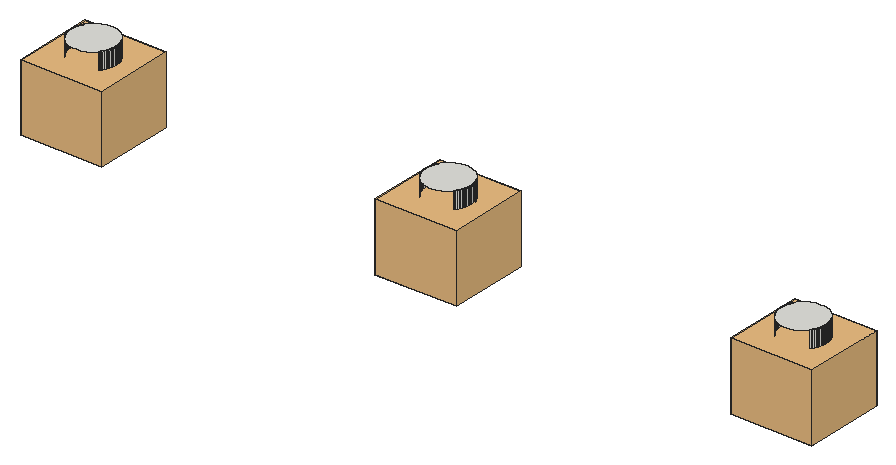
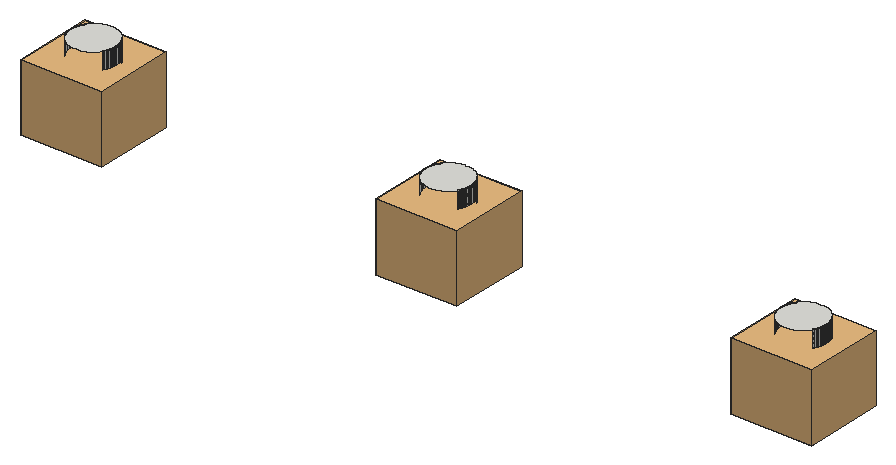
# SketchUp Ruby script. Lengths in inches.
U = 1.inch
M = Sketchup.active_model
def pt(a) = Geom::Point3d.new(a.map { |v| v * U })
def face(e, loops, mat)
  f = e.add_face(loops[0].map { |a| pt(a) })
  loops[1..].each { |l| e.add_face(l.map { |a| pt(a) }).erase! }
  f.material = f.back_material = mat if mat
  f
end
# faces: each face lists its corners as indices into pts; further lists are holes
def faces(e, pts, list, mat = nil) = list.each { |f| face(e, (f[0].is_a?(Array) ? f : [f]).map { |l| l.map { |i| pts[i] } }, mat) }
# xy, xz, yz: faces in a plane at the given z, y or x. An outline is a flat list of corners, or four numbers for a rectangle; further outlines are holes
def ring(l) = l.size == 4 ? [[l[0], l[1]], [l[2], l[1]], [l[2], l[3]], [l[0], l[3]]] : l.each_slice(2).to_a
def flat(e, list, mat, &to3) = list.each { |f| face(e, (f[0].is_a?(Array) ? f : [f]).map { |l| ring(l).map { |u, v| to3.(u, v) } }, mat) }
def xy(e, z, list, mat = nil) = flat(e, list, mat) { |x, y| [x, y, z] }
def xz(e, y, list, mat = nil) = flat(e, list, mat) { |x, z| [x, y, z] }
def yz(e, x, list, mat = nil) = flat(e, list, mat) { |y, z| [x, y, z] }
def lines(e, pts, list) = list.each { |a, b| e.add_line(pt(pts[a]), pt(pts[b])) }
# prism: a flat outline (further loops are holes) pulled along v
def prism(e, loops, v, mat = nil)
  f = face(e, loops, mat); d = Geom::Vector3d.new(v.map { |x| x * U })
  f.pushpull(f.normal.samedirection?(d) ? d.length : -d.length)
end
def box(e, o, s, mat = nil) = prism(e, [[o, [o[0] + s[0], o[1], o[2]], [o[0] + s[0], o[1] + s[1], o[2]], [o[0], o[1] + s[1], o[2]]]], [0, 0, s[2]], mat)
def at(x, y, z, deg = 0) = Geom::Transformation.translation(pt([x, y, z])) * Geom::Transformation.rotation(ORIGIN, Z_AXIS, deg.degrees)
def axes(o, x, y, z) = Geom::Transformation.new([*x, 0, *y, 0, *z, 0, *pt(o).to_a, 1])
def part(name) = M.definitions.add(name)
# library, detail: a bought-in or finely detailed component or shape, given as its bounding box
def library(name, o, s) = part(name).tap { |d| box(d.entities, o, s) }
def detail(e, o, s) = box(e.add_group.entities, o, s)
def put(e, d, t, mat = nil) = e.add_instance(d, t).tap { |i| i.material = mat if mat }
def group(e, t, mat = nil) = e.add_group.tap { |g| g.transformation = t; g.material = mat if mat }.entities
root = M.entities
c1 = library("2",[-3.42,-3.42,-12.15],[10.84,10.84,12.15])
xy(root,250,[[55.9,272.75,55.66,272.78,55.59,272.79,55.51,272.8,55.43,272.82,55.35,272.83,55.28,272.85,55.2,272.875,55.13,272.9,55.05,272.92,54.91,272.98,54.83,273.01,54.76,273.04,54.69,273.08,54.625,273.11,54.55,273.15,54.49,273.19,54.42,273.23,54.36,273.28,54.29,273.32,53.99,273.57,53.88,273.68,53.83,273.74,53.77,273.8,53.67,273.92,53.63,273.99,53.58,274.05,53.54,274.12,53.5,274.18,53.38,274.39,53.35,274.46,53.3125,274.53,53.28,274.6,53.25,274.67,53.23,274.75,53.2,274.82,53.18,274.9,53.16,274.97,53.14,275.05,53.12,275.125,53.11,275.2,53.09,275.28,53.08,275.36,53.07,275.4375,53.0625,275.51,53.06,275.59,53.06,275.67,53.05,275.75,53.06,275.83,53.06,275.91,53.0625,275.99,53.07,276.0625,53.08,276.14,53.09,276.22,53.11,276.3,53.12,276.375,53.14,276.45,53.16,276.53,53.18,276.6,53.2,276.68,53.23,276.75,53.25,276.83,53.28,276.9,53.3125,276.97,53.35,277.04,53.38,277.11,53.5,277.32,53.54,277.38,53.58,277.45,53.63,277.51,53.67,277.58,53.77,277.7,53.83,277.76,53.88,277.82,53.99,277.93,54.29,278.18,54.36,278.22,54.42,278.27,54.49,278.31,54.55,278.35,54.625,278.39,54.69,278.42,54.76,278.46,54.83,278.49,54.91,278.52,55.05,278.58,55.13,278.6,55.2,278.625,55.28,278.65,55.35,278.67,55.43,278.68,55.51,278.7,55.59,278.71,55.66,278.72,55.9,278.75,56.21,278.75,56.45,278.72,56.52,278.71,56.6,278.7,56.68,278.68,56.76,278.67,56.83,278.65,56.91,278.625,56.98,278.6,57.06,278.58,57.27,278.49,57.35,278.46,57.42,278.42,57.49,278.39,57.55,278.35,57.62,278.31,57.6875,278.27,57.75,278.22,57.82,278.18,58,278.03,58.0625,277.98,58.12,277.93,58.23,277.82,58.28,277.76,58.34,277.7,58.39,277.64,58.43,277.58,58.48,277.51,58.53,277.45,58.57,277.38,58.61,277.32,58.73,277.11,58.76,277.04,58.8,276.97,58.86,276.83,58.88,276.75,58.91,276.68,58.93,276.6,58.95,276.53,58.97,276.45,58.99,276.375,59,276.3,59.02,276.22,59.03,276.14,59.04,276.0625,59.05,275.99,59.05,275.51,59.04,275.4375,59.03,275.36,59.02,275.28,59,275.2,58.99,275.125,58.97,275.05,58.95,274.97,58.93,274.9,58.91,274.82,58.88,274.75,58.86,274.67,58.8,274.53,58.76,274.46,58.73,274.39,58.61,274.18,58.57,274.12,58.53,274.05,58.48,273.99,58.43,273.92,58.39,273.86,58.34,273.8,58.28,273.74,58.23,273.68,58.12,273.57,58.0625,273.52,58,273.47,57.82,273.32,57.75,273.28,57.6875,273.23,57.62,273.19,57.55,273.15,57.49,273.11,57.42,273.08,57.35,273.04,57.27,273.01,57.06,272.92,56.98,272.9,56.91,272.875,56.83,272.85,56.76,272.83,56.68,272.82,56.6,272.8,56.52,272.79,56.45,272.78,56.21,272.75],[103.34,272.75,103.26,272.76,103.1875,272.77,103.11,272.78,102.95,272.8,102.875,272.82,102.8,272.83,102.72,272.85,102.65,272.875,102.57,272.9,102.5,272.92,102.42,272.95,102.21,273.04,102.14,273.08,102.07,273.11,101.93,273.19,101.87,273.23,101.8,273.28,101.74,273.32,101.67,273.37,101.43,273.57,101.38,273.63,101.32,273.68,101.12,273.92,101.07,273.99,101.03,274.05,100.98,274.12,100.94,274.18,100.86,274.32,100.83,274.39,100.79,274.46,100.7,274.67,100.67,274.75,100.65,274.82,100.625,274.9,100.6,274.97,100.58,275.05,100.57,275.125,100.55,275.2,100.53,275.36,100.52,275.4375,100.51,275.51,100.5,275.59,100.5,275.91,100.51,275.99,100.52,276.0625,100.53,276.14,100.55,276.3,100.57,276.375,100.58,276.45,100.6,276.53,100.625,276.6,100.65,276.68,100.67,276.75,100.7,276.83,100.79,277.04,100.83,277.11,100.86,277.18,100.94,277.32,100.98,277.38,101.03,277.45,101.07,277.51,101.12,277.58,101.32,277.82,101.38,277.87,101.43,277.93,101.67,278.13,101.74,278.18,101.8,278.22,101.87,278.27,101.93,278.31,102.07,278.39,102.14,278.42,102.21,278.46,102.42,278.55,102.5,278.58,102.57,278.6,102.65,278.625,102.72,278.65,102.8,278.67,102.875,278.68,102.95,278.7,103.11,278.72,103.1875,278.73,103.26,278.74,103.34,278.75,103.66,278.75,103.74,278.74,103.8125,278.73,103.89,278.72,104.05,278.7,104.125,278.68,104.2,278.67,104.28,278.65,104.35,278.625,104.43,278.6,104.5,278.58,104.58,278.55,104.79,278.46,104.86,278.42,104.93,278.39,105.07,278.31,105.13,278.27,105.2,278.22,105.26,278.18,105.33,278.13,105.57,277.93,105.62,277.87,105.68,277.82,105.88,277.58,105.93,277.51,105.97,277.45,106.02,277.38,106.06,277.32,106.14,277.18,106.17,277.11,106.21,277.04,106.3,276.83,106.33,276.75,106.35,276.68,106.375,276.6,106.4,276.53,106.42,276.45,106.43,276.375,106.45,276.3,106.47,276.14,106.48,276.0625,106.49,275.99,106.5,275.91,106.5,275.59,106.49,275.51,106.48,275.4375,106.47,275.36,106.45,275.2,106.43,275.125,106.42,275.05,106.4,274.97,106.375,274.9,106.35,274.82,106.33,274.75,106.3,274.67,106.21,274.46,106.17,274.39,106.14,274.32,106.06,274.18,106.02,274.12,105.97,274.05,105.93,273.99,105.88,273.92,105.68,273.68,105.62,273.63,105.57,273.57,105.33,273.37,105.26,273.32,105.2,273.28,105.13,273.23,105.07,273.19,104.93,273.11,104.86,273.08,104.79,273.04,104.58,272.95,104.5,272.92,104.43,272.9,104.35,272.875,104.28,272.85,104.2,272.83,104.125,272.82,104.05,272.8,103.89,272.78,103.8125,272.77,103.74,272.76,103.66,272.75],[150.79,272.75,150.55,272.78,150.48,272.79,150.4,272.8,150.32,272.82,150.24,272.83,150.17,272.85,150.09,272.875,150.02,272.9,149.94,272.92,149.73,273.01,149.65,273.04,149.58,273.08,149.51,273.11,149.45,273.15,149.38,273.19,149.3125,273.23,149.25,273.28,149.18,273.32,149,273.47,148.9375,273.52,148.88,273.57,148.77,273.68,148.72,273.74,148.66,273.8,148.61,273.86,148.57,273.92,148.52,273.99,148.47,274.05,148.43,274.12,148.39,274.18,148.27,274.39,148.24,274.46,148.2,274.53,148.14,274.67,148.12,274.75,148.09,274.82,148.07,274.9,148.05,274.97,148.03,275.05,148.01,275.125,148,275.2,147.98,275.28,147.97,275.36,147.96,275.4375,147.95,275.51,147.95,275.99,147.96,276.0625,147.97,276.14,147.98,276.22,148,276.3,148.01,276.375,148.03,276.45,148.05,276.53,148.07,276.6,148.09,276.68,148.12,276.75,148.14,276.83,148.2,276.97,148.24,277.04,148.27,277.11,148.39,277.32,148.43,277.38,148.47,277.45,148.52,277.51,148.57,277.58,148.61,277.64,148.66,277.7,148.72,277.76,148.77,277.82,148.88,277.93,148.9375,277.98,149,278.03,149.18,278.18,149.25,278.22,149.3125,278.27,149.38,278.31,149.45,278.35,149.51,278.39,149.58,278.42,149.65,278.46,149.73,278.49,149.94,278.58,150.02,278.6,150.09,278.625,150.17,278.65,150.24,278.67,150.32,278.68,150.4,278.7,150.48,278.71,150.55,278.72,150.79,278.75,151.1,278.75,151.34,278.72,151.41,278.71,151.49,278.7,151.57,278.68,151.65,278.67,151.72,278.65,151.8,278.625,151.87,278.6,151.95,278.58,152.09,278.52,152.17,278.49,152.24,278.46,152.31,278.42,152.375,278.39,152.45,278.35,152.51,278.31,152.58,278.27,152.64,278.22,152.71,278.18,153.01,277.93,153.12,277.82,153.17,277.76,153.23,277.7,153.33,277.58,153.37,277.51,153.42,277.45,153.46,277.38,153.5,277.32,153.62,277.11,153.65,277.04,153.6875,276.97,153.72,276.9,153.75,276.83,153.77,276.75,153.8,276.68,153.82,276.6,153.84,276.53,153.86,276.45,153.88,276.375,153.89,276.3,153.91,276.22,153.92,276.14,153.93,276.0625,153.9375,275.99,153.94,275.91,153.94,275.83,153.95,275.75,153.94,275.67,153.94,275.59,153.9375,275.51,153.93,275.4375,153.92,275.36,153.91,275.28,153.89,275.2,153.88,275.125,153.86,275.05,153.84,274.97,153.82,274.9,153.8,274.82,153.77,274.75,153.75,274.67,153.72,274.6,153.6875,274.53,153.65,274.46,153.62,274.39,153.5,274.18,153.46,274.12,153.42,274.05,153.37,273.99,153.33,273.92,153.23,273.8,153.17,273.74,153.12,273.68,153.01,273.57,152.71,273.32,152.64,273.28,152.58,273.23,152.51,273.19,152.45,273.15,152.375,273.11,152.31,273.08,152.24,273.04,152.17,273.01,152.09,272.98,151.95,272.92,151.87,272.9,151.8,272.875,151.72,272.85,151.65,272.83,151.57,272.82,151.49,272.8,151.41,272.79,151.34,272.78,151.1,272.75]])
yz(root,53.06,[[275.59,247,275.67,250],[275.83,247,275.91,250]])
yz(root,59.05,[[275.51,247,275.59,250],[275.59,247,275.67,250],[275.67,247,275.75,250],[275.75,247,275.83,250],[275.83,247,275.91,250],
  [275.91,247,275.99,250]])
yz(root,100.5,[[275.59,247,275.67,250],[275.67,247,275.75,250],[275.75,247,275.83,250],[275.83,247,275.91,250]])
yz(root,106.5,[[275.59,247,275.67,250],[275.67,247,275.75,250],[275.75,247,275.83,250],[275.83,247,275.91,250]])
yz(root,147.95,[[275.51,247,275.59,250],[275.59,247,275.67,250],[275.67,247,275.75,250],[275.75,247,275.83,250],[275.83,247,275.91,250],
  [275.91,247,275.99,250]])
yz(root,153.94,[[275.59,247,275.67,250],[275.83,247,275.91,250]])
p = [[58.39,273.86,250],[58.39,273.86,247],[58.34,273.8,247],[58.34,273.8,250],[105.83,273.86,250],[105.83,273.86,247],
  [105.78,273.8,247],[105.78,273.8,250],[53.67,273.92,250],[53.67,273.92,247],[53.63,273.99,247],[53.63,273.99,250],
  [53.72,273.86,250],[53.72,273.86,247],[58.43,273.92,250],[58.43,273.92,247],[58.48,273.99,250],[58.48,273.99,247],
  [101.17,273.86,250],[101.17,273.86,247],[101.12,273.92,247],[101.12,273.92,250],[101.07,273.99,247],[101.07,273.99,250],
  [105.88,273.92,250],[105.88,273.92,247],[105.93,273.99,250],[105.93,273.99,247],[148.57,273.92,250],[148.57,273.92,247],
  [148.52,273.99,247],[148.52,273.99,250],[148.61,273.86,250],[148.61,273.86,247],[153.33,273.92,250],[153.33,273.92,247],
  [153.28,273.86,247],[153.28,273.86,250],[153.37,273.99,250],[153.37,273.99,247],[53.58,274.05,247],[53.58,274.05,250],
  [58.53,274.05,250],[58.53,274.05,247],[101.03,274.05,247],[101.03,274.05,250],[105.97,274.05,250],[105.97,274.05,247],
  [148.47,274.05,247],[148.47,274.05,250],[153.42,274.05,250],[153.42,274.05,247],[53.54,274.12,247],[53.54,274.12,250],
  [53.5,274.18,247],[53.5,274.18,250],[58.57,274.12,250],[58.57,274.12,247],[58.61,274.18,250],[58.61,274.18,247],
  [100.98,274.12,250],[100.98,274.12,247],[100.94,274.18,247],[100.94,274.18,250],[106.02,274.12,250],[106.02,274.12,247],
  [106.06,274.18,250],[106.06,274.18,247],[148.43,274.12,247],[148.43,274.12,250],[148.39,274.18,247],[148.39,274.18,250],
  [153.46,274.12,250],[153.46,274.12,247],[153.5,274.18,250],[153.5,274.18,247],[53.46,274.25,247],[53.46,274.25,250],
  [58.65,274.25,250],[58.65,274.25,247],[100.9,274.25,247],[100.9,274.25,250],[106.1,274.25,250],[106.1,274.25,247],
  [148.35,274.25,247],[148.35,274.25,250],[153.54,274.25,250],[153.54,274.25,247],[53.42,274.32,247],[53.42,274.32,250],
  [53.38,274.39,247],[53.38,274.39,250],[58.69,274.32,250],[58.69,274.32,247],[58.73,274.39,250],[58.73,274.39,247],
  [100.86,274.32,250],[100.86,274.32,247],[100.83,274.39,247],[100.83,274.39,250],[106.14,274.32,250],[106.14,274.32,247],
  [106.17,274.39,250],[106.17,274.39,247],[148.31,274.32,247],[148.31,274.32,250],[148.27,274.39,247],[148.27,274.39,250],
  [153.58,274.32,250],[153.58,274.32,247],[153.62,274.39,250],[153.62,274.39,247],[53.35,274.46,247],[53.35,274.46,250],
  [58.76,274.46,250],[58.76,274.46,247],[100.79,274.46,247],[100.79,274.46,250],[106.21,274.46,250],[106.21,274.46,247],
  [148.24,274.46,247],[148.24,274.46,250],[153.65,274.46,250],[153.65,274.46,247],[53.3125,274.53,247],[53.3125,274.53,250],
  [53.28,274.6,247],[53.28,274.6,250],[58.8,274.53,250],[58.8,274.53,247],[58.83,274.6,250],[58.83,274.6,247],
  [100.76,274.53,250],[100.76,274.53,247],[100.73,274.6,247],[100.73,274.6,250],[106.24,274.53,250],[106.24,274.53,247],
  [106.27,274.6,250],[106.27,274.6,247],[148.2,274.53,247],[148.2,274.53,250],[148.17,274.6,247],[148.17,274.6,250],
  [153.6875,274.53,250],[153.6875,274.53,247],[153.72,274.6,250],[153.72,274.6,247],[53.25,274.67,247],[53.25,274.67,250],
  [58.86,274.67,250],[58.86,274.67,247],[100.7,274.67,247],[100.7,274.67,250],[106.3,274.67,250],[106.3,274.67,247],
  [148.14,274.67,247],[148.14,274.67,250],[153.75,274.67,250],[153.75,274.67,247],[53.23,274.75,247],[53.23,274.75,250],
  [53.2,274.82,247],[53.2,274.82,250],[58.88,274.75,250],[58.88,274.75,247],[58.91,274.82,250],[58.91,274.82,247],
  [100.67,274.75,250],[100.67,274.75,247],[100.65,274.82,247],[100.65,274.82,250],[106.33,274.75,250],[106.33,274.75,247],
  [106.35,274.82,250],[106.35,274.82,247],[148.12,274.75,247],[148.12,274.75,250],[148.09,274.82,247],[148.09,274.82,250],
  [153.77,274.75,250],[153.77,274.75,247],[153.8,274.82,250],[153.8,274.82,247],[53.18,274.9,247],[53.18,274.9,250],
  [58.93,274.9,250],[58.93,274.9,247],[100.625,274.9,247],[100.625,274.9,250],[106.375,274.9,250],[106.375,274.9,247],
  [148.07,274.9,247],[148.07,274.9,250],[153.82,274.9,250],[153.82,274.9,247],[53.16,274.97,247],[53.16,274.97,250],
  [58.95,274.97,250],[58.95,274.97,247],[100.6,274.97,247],[100.6,274.97,250],[106.4,274.97,250],[106.4,274.97,247],
  [148.05,274.97,247],[148.05,274.97,250],[153.84,274.97,250],[153.84,274.97,247],[53.14,275.05,247],[53.14,275.05,250],
  [53.12,275.125,247],[53.12,275.125,250],[58.97,275.05,250],[58.97,275.05,247],[58.99,275.125,250],[58.99,275.125,247],
  [100.58,275.05,247],[100.58,275.05,250],[100.57,275.125,247],[100.57,275.125,250],[106.42,275.05,250],[106.42,275.05,247],
  [106.43,275.125,250],[106.43,275.125,247],[148.03,275.05,247],[148.03,275.05,250],[148.01,275.125,247],[148.01,275.125,250],
  [153.86,275.05,250],[153.86,275.05,247],[153.88,275.125,250],[153.88,275.125,247],[53.11,275.2,247],[53.11,275.2,250],
  [59,275.2,250],[59,275.2,247],[100.55,275.2,247],[100.55,275.2,250],[106.45,275.2,250],[106.45,275.2,247],
  [148,275.2,247],[148,275.2,250],[153.89,275.2,250],[153.89,275.2,247],[53.09,275.28,247],[53.09,275.28,250],
  [59.02,275.28,250],[59.02,275.28,247],[100.54,275.28,247],[100.54,275.28,250],[106.46,275.28,250],[106.46,275.28,247],
  [147.98,275.28,247],[147.98,275.28,250],[153.91,275.28,250],[153.91,275.28,247],[53.08,275.36,247],[53.08,275.36,250],
  [59.03,275.36,250],[59.03,275.36,247],[100.53,275.36,247],[100.53,275.36,250],[106.47,275.36,250],[106.47,275.36,247],
  [147.97,275.36,247],[147.97,275.36,250],[153.92,275.36,250],[153.92,275.36,247],[53.07,275.4375,247],[53.07,275.4375,250],
  [53.0625,275.51,247],[53.0625,275.51,250],[59.04,275.4375,250],[59.04,275.4375,247],[59.05,275.51,250],[59.05,275.51,247],
  [100.52,275.4375,247],[100.52,275.4375,250],[100.51,275.51,247],[100.51,275.51,250],[106.48,275.4375,250],[106.48,275.4375,247],
  [106.49,275.51,250],[106.49,275.51,247],[147.96,275.4375,247],[147.96,275.4375,250],[147.95,275.51,247],[147.95,275.51,250],
  [153.93,275.4375,250],[153.93,275.4375,247],[153.9375,275.51,250],[153.9375,275.51,247],[53.06,275.59,247],[53.06,275.59,250],
  [100.5,275.59,247],[100.5,275.59,250],[106.5,275.59,250],[106.5,275.59,247],[153.94,275.59,250],[153.94,275.59,247],
  [53.06,275.67,250],[53.06,275.67,247],[53.05,275.75,247],[53.05,275.75,250],[153.95,275.75,250],[153.95,275.75,247],
  [153.94,275.67,247],[153.94,275.67,250],[53.06,275.83,247],[53.06,275.83,250],[153.94,275.83,250],[153.94,275.83,247],
  [53.06,275.91,250],[53.06,275.91,247],[53.0625,275.99,247],[53.0625,275.99,250],[100.5,275.91,250],[100.5,275.91,247],
  [100.51,275.99,247],[100.51,275.99,250],[106.49,275.99,250],[106.49,275.99,247],[106.5,275.91,247],[106.5,275.91,250],
  [153.9375,275.99,250],[153.9375,275.99,247],[153.94,275.91,247],[153.94,275.91,250],[53.07,276.0625,247],[53.07,276.0625,250],
  [59.04,276.0625,250],[59.04,276.0625,247],[59.05,275.99,247],[59.05,275.99,250],[100.52,276.0625,247],[100.52,276.0625,250],
  [106.48,276.0625,250],[106.48,276.0625,247],[147.95,275.99,250],[147.95,275.99,247],[147.96,276.0625,247],[147.96,276.0625,250],
  [153.93,276.0625,250],[153.93,276.0625,247],[53.08,276.14,247],[53.08,276.14,250],[53.09,276.22,247],[53.09,276.22,250],
  [59.03,276.14,250],[59.03,276.14,247],[59.02,276.22,250],[59.02,276.22,247],[100.53,276.14,247],[100.53,276.14,250],
  [100.54,276.22,247],[100.54,276.22,250],[106.47,276.14,250],[106.47,276.14,247],[106.46,276.22,250],[106.46,276.22,247],
  [147.97,276.14,247],[147.97,276.14,250],[147.98,276.22,247],[147.98,276.22,250],[153.92,276.14,250],[153.92,276.14,247],
  [153.91,276.22,250],[153.91,276.22,247],[53.11,276.3,247],[53.11,276.3,250],[59,276.3,250],[59,276.3,247],
  [100.55,276.3,247],[100.55,276.3,250],[106.45,276.3,250],[106.45,276.3,247],[148,276.3,247],[148,276.3,250],
  [153.89,276.3,250],[153.89,276.3,247],[53.12,276.375,247],[53.12,276.375,250],[58.99,276.375,250],[58.99,276.375,247],
  [100.57,276.375,247],[100.57,276.375,250],[106.43,276.375,250],[106.43,276.375,247],[148.01,276.375,247],[148.01,276.375,250],
  [153.88,276.375,250],[153.88,276.375,247],[53.14,276.45,247],[53.14,276.45,250],[58.97,276.45,250],[58.97,276.45,247],
  [100.58,276.45,247],[100.58,276.45,250],[106.42,276.45,250],[106.42,276.45,247],[148.03,276.45,247],[148.03,276.45,250],
  [153.86,276.45,250],[153.86,276.45,247],[53.16,276.53,247],[53.16,276.53,250],[53.18,276.6,247],[53.18,276.6,250],
  [58.93,276.6,250],[58.93,276.6,247],[58.95,276.53,247],[58.95,276.53,250],[100.6,276.53,247],[100.6,276.53,250],
  [100.625,276.6,247],[100.625,276.6,250],[106.4,276.53,250],[106.4,276.53,247],[106.375,276.6,250],[106.375,276.6,247],
  [148.05,276.53,247],[148.05,276.53,250],[148.07,276.6,247],[148.07,276.6,250],[153.84,276.53,250],[153.84,276.53,247],
  [153.82,276.6,250],[153.82,276.6,247],[53.2,276.68,247],[53.2,276.68,250],[58.91,276.68,250],[58.91,276.68,247],
  [100.65,276.68,247],[100.65,276.68,250],[106.35,276.68,250],[106.35,276.68,247],[148.09,276.68,247],[148.09,276.68,250],
  [153.8,276.68,250],[153.8,276.68,247],[53.23,276.75,247],[53.23,276.75,250],[58.88,276.75,250],[58.88,276.75,247],
  [100.67,276.75,247],[100.67,276.75,250],[106.33,276.75,250],[106.33,276.75,247],[148.12,276.75,247],[148.12,276.75,250],
  [153.77,276.75,250],[153.77,276.75,247],[53.25,276.83,247],[53.25,276.83,250],[53.28,276.9,247],[53.28,276.9,250],
  [58.83,276.9,250],[58.83,276.9,247],[58.86,276.83,247],[58.86,276.83,250],[100.7,276.83,247],[100.7,276.83,250],
  [100.73,276.9,247],[100.73,276.9,250],[106.3,276.83,250],[106.3,276.83,247],[106.27,276.9,250],[106.27,276.9,247],
  [148.14,276.83,247],[148.14,276.83,250],[148.17,276.9,247],[148.17,276.9,250],[153.75,276.83,250],[153.75,276.83,247],
  [153.72,276.9,250],[153.72,276.9,247],[53.3125,276.97,247],[53.3125,276.97,250],[58.8,276.97,250],[58.8,276.97,247],
  [100.76,276.97,247],[100.76,276.97,250],[106.24,276.97,250],[106.24,276.97,247],[148.2,276.97,247],[148.2,276.97,250],
  [153.6875,276.97,250],[153.6875,276.97,247],[53.35,277.04,247],[53.35,277.04,250],[53.38,277.11,247],[53.38,277.11,250],
  [58.73,277.11,250],[58.73,277.11,247],[58.76,277.04,247],[58.76,277.04,250],[100.79,277.04,247],[100.79,277.04,250],
  [100.83,277.11,247],[100.83,277.11,250],[106.21,277.04,250],[106.21,277.04,247],[106.17,277.11,250],[106.17,277.11,247],
  [148.24,277.04,247],[148.24,277.04,250],[148.27,277.11,247],[148.27,277.11,250],[153.62,277.11,250],[153.62,277.11,247],
  [153.65,277.04,247],[153.65,277.04,250],[53.42,277.18,247],[53.42,277.18,250],[58.69,277.18,250],[58.69,277.18,247],
  [100.86,277.18,247],[100.86,277.18,250],[106.14,277.18,250],[106.14,277.18,247],[148.31,277.18,247],[148.31,277.18,250],
  [153.58,277.18,250],[153.58,277.18,247],[53.46,277.25,247],[53.46,277.25,250],[58.65,277.25,250],[58.65,277.25,247],
  [100.9,277.25,247],[100.9,277.25,250],[106.1,277.25,250],[106.1,277.25,247],[148.35,277.25,247],[148.35,277.25,250],
  [153.54,277.25,250],[153.54,277.25,247],[53.5,277.32,247],[53.5,277.32,250],[100.94,277.32,247],[100.94,277.32,250],
  [106.06,277.32,250],[106.06,277.32,247],[148.39,277.32,247],[148.39,277.32,250],[153.5,277.32,250],[153.5,277.32,247]]
faces(root,p,[[0,1,2,3],[4,5,6,7],[8,9,10,11],[12,13,9,8],[14,15,1,0],[16,17,15,14],[18,19,20,21],[21,20,22,23],
  [24,25,5,4],[26,27,25,24],[28,29,30,31],[32,33,29,28],[34,35,36,37],[38,39,35,34],[11,10,40,41],[42,43,17,16],
  [23,22,44,45],[46,47,27,26],[31,30,48,49],[50,51,39,38],[41,40,52,53],[53,52,54,55],[56,57,43,42],[58,59,57,56],
  [60,61,62,63],[45,44,61,60],[64,65,47,46],[66,67,65,64],[49,48,68,69],[69,68,70,71],[72,73,51,50],[74,75,73,72],
  [55,54,76,77],[78,79,59,58],[63,62,80,81],[82,83,67,66],[71,70,84,85],[86,87,75,74],[77,76,88,89],[89,88,90,91],
  [92,93,79,78],[94,95,93,92],[96,97,98,99],[81,80,97,96],[100,101,83,82],[102,103,101,100],[85,84,104,105],[105,104,106,107],
  [108,109,87,86],[110,111,109,108],[91,90,112,113],[114,115,95,94],[99,98,116,117],[118,119,103,102],[107,106,120,121],[122,123,111,110],
  [113,112,124,125],[125,124,126,127],[128,129,115,114],[130,131,129,128],[132,133,134,135],[117,116,133,132],[136,137,119,118],[138,139,137,136],
  [121,120,140,141],[141,140,142,143],[144,145,123,122],[146,147,145,144],[127,126,148,149],[150,151,131,130],[135,134,152,153],[154,155,139,138],
  [143,142,156,157],[158,159,147,146],[149,148,160,161],[161,160,162,163],[164,165,151,150],[166,167,165,164],[168,169,170,171],[153,152,169,168],
  [172,173,155,154],[174,175,173,172],[157,156,176,177],[177,176,178,179],[180,181,159,158],[182,183,181,180],[163,162,184,185],[186,187,167,166],
  [171,170,188,189],[190,191,175,174],[179,178,192,193],[194,195,183,182],[185,184,196,197],[198,199,187,186],[189,188,200,201],[202,203,191,190],
  [193,192,204,205],[206,207,195,194],[197,196,208,209],[209,208,210,211],[212,213,199,198],[214,215,213,212],[201,200,216,217],[217,216,218,219],
  [220,221,203,202],[222,223,221,220],[205,204,224,225],[225,224,226,227],[228,229,207,206],[230,231,229,228],[211,210,232,233],[234,235,215,214],
  [219,218,236,237],[238,239,223,222],[227,226,240,241],[242,243,231,230],[233,232,244,245],[246,247,235,234],[237,236,248,249],[250,251,239,238],
  [241,240,252,253],[254,255,243,242],[245,244,256,257],[258,259,247,246],[249,248,260,261],[262,263,251,250],[253,252,264,265],[266,267,255,254],
  [257,256,268,269],[269,268,270,271],[272,273,259,258],[274,275,273,272],[261,260,276,277],[277,276,278,279],[280,281,263,262],[282,283,281,280],
  [265,264,284,285],[285,284,286,287],[288,289,267,266],[290,291,289,288],[271,270,292,293],[279,278,294,295],[296,297,283,282],[298,299,291,290],
  [300,301,302,303],[304,305,306,307],[303,302,308,309],[310,311,305,304],[312,313,314,315],[316,317,318,319],[320,321,322,323],[324,325,326,327],
  [315,314,328,329],[330,331,332,333],[319,318,334,335],[336,337,321,320],[338,339,340,341],[342,343,325,324],[329,328,344,345],[345,344,346,347],
  [348,349,331,330],[350,351,349,348],[335,334,352,353],[353,352,354,355],[356,357,337,336],[358,359,357,356],[341,340,360,361],[361,360,362,363],
  [364,365,343,342],[366,367,365,364],[347,346,368,369],[370,371,351,350],[355,354,372,373],[374,375,359,358],[363,362,376,377],[378,379,367,366],
  [369,368,380,381],[382,383,371,370],[373,372,384,385],[386,387,375,374],[377,376,388,389],[390,391,379,378],[381,380,392,393],[394,395,383,382],
  [385,384,396,397],[398,399,387,386],[389,388,400,401],[402,403,391,390],[393,392,404,405],[405,404,406,407],[408,409,410,411],[411,410,395,394],
  [397,396,412,413],[413,412,414,415],[416,417,399,398],[418,419,417,416],[401,400,420,421],[421,420,422,423],[424,425,403,402],[426,427,425,424],
  [407,406,428,429],[430,431,409,408],[415,414,432,433],[434,435,419,418],[423,422,436,437],[438,439,427,426],[429,428,440,441],[442,443,431,430],
  [433,432,444,445],[446,447,435,434],[437,436,448,449],[450,451,439,438],[441,440,452,453],[453,452,454,455],[456,457,458,459],[459,458,443,442],
  [445,444,460,461],[461,460,462,463],[464,465,447,446],[466,467,465,464],[449,448,468,469],[469,468,470,471],[472,473,451,450],[474,475,473,472],
  [455,454,476,477],[478,479,457,456],[463,462,480,481],[482,483,467,466],[471,470,484,485],[486,487,475,474],[477,476,488,489],[489,488,490,491],
  [492,493,494,495],[495,494,479,478],[481,480,496,497],[497,496,498,499],[500,501,483,482],[502,503,501,500],[485,484,504,505],[505,504,506,507],
  [508,509,510,511],[511,510,487,486],[491,490,512,513],[514,515,493,492],[499,498,516,517],[518,519,503,502],[507,506,520,521],[522,523,509,508],
  [513,512,524,525],[526,527,515,514],[517,516,528,529],[530,531,519,518],[521,520,532,533],[534,535,523,522],[525,524,536,537],[529,528,538,539],
  [540,541,531,530],[533,532,542,543],[544,545,535,534]])
put(root,c1,axes([54.06,273.75,247.81],[1,0,0],[0,1,0],[0,0,0.7425]))
put(root,c1,axes([101.5,273.75,247.81],[1,0,0],[0,1,0],[0,0,0.7425]))
put(root,c1,axes([148.95,273.75,247.81],[1,0,0],[0,1,0],[0,0,0.7425]))
